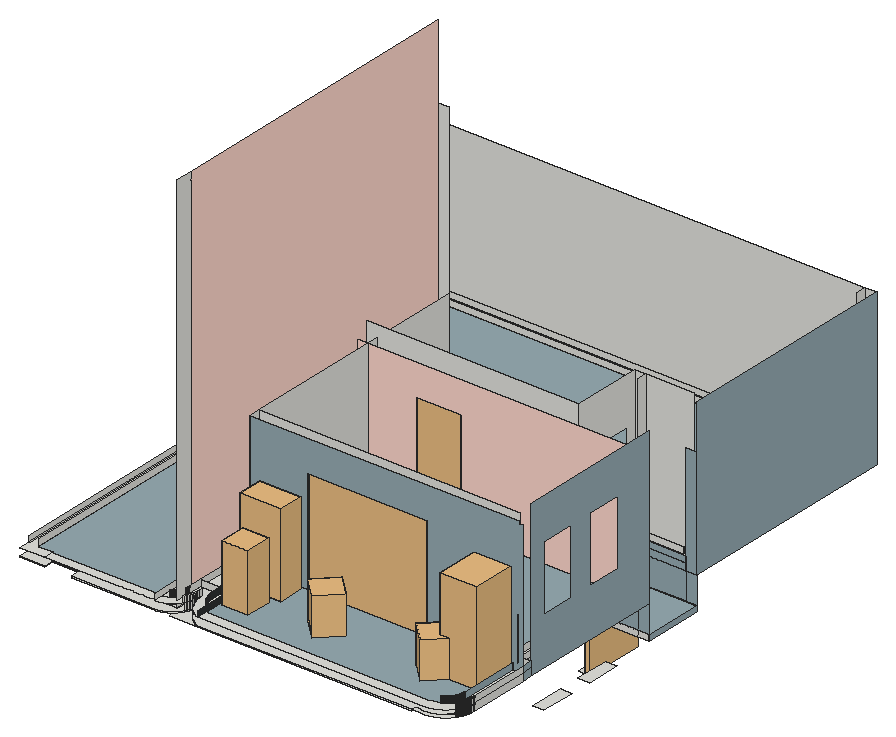
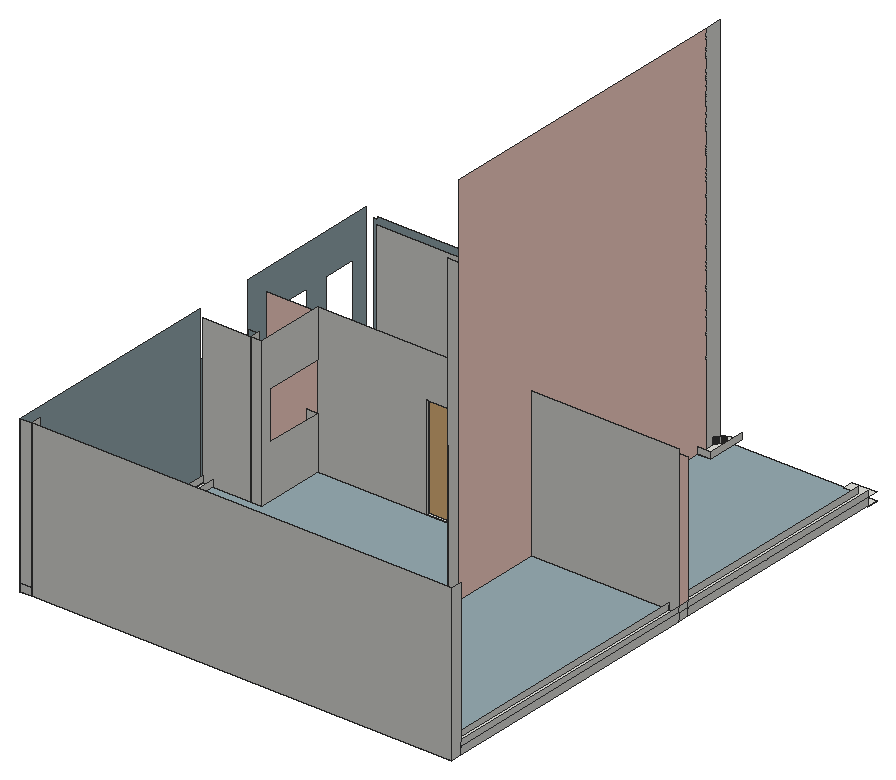
# SketchUp Ruby script. Lengths in inches.
U = 1.inch
M = Sketchup.active_model
def pt(a) = Geom::Point3d.new(a.map { |v| v * U })
def face(e, loops, mat)
  f = e.add_face(loops[0].map { |a| pt(a) })
  loops[1..].each { |l| e.add_face(l.map { |a| pt(a) }).erase! }
  f.material = f.back_material = mat if mat
  f
end
# faces: each face lists its corners as indices into pts; further lists are holes
def faces(e, pts, list, mat = nil) = list.each { |f| face(e, (f[0].is_a?(Array) ? f : [f]).map { |l| l.map { |i| pts[i] } }, mat) }
# xy, xz, yz: faces in a plane at the given z, y or x. An outline is a flat list of corners, or four numbers for a rectangle; further outlines are holes
def ring(l) = l.size == 4 ? [[l[0], l[1]], [l[2], l[1]], [l[2], l[3]], [l[0], l[3]]] : l.each_slice(2).to_a
def flat(e, list, mat, &to3) = list.each { |f| face(e, (f[0].is_a?(Array) ? f : [f]).map { |l| ring(l).map { |u, v| to3.(u, v) } }, mat) }
def xy(e, z, list, mat = nil) = flat(e, list, mat) { |x, y| [x, y, z] }
def xz(e, y, list, mat = nil) = flat(e, list, mat) { |x, z| [x, y, z] }
def yz(e, x, list, mat = nil) = flat(e, list, mat) { |y, z| [x, y, z] }
def lines(e, pts, list) = list.each { |a, b| e.add_line(pt(pts[a]), pt(pts[b])) }
# prism: a flat outline (further loops are holes) pulled along v
def prism(e, loops, v, mat = nil)
  f = face(e, loops, mat); d = Geom::Vector3d.new(v.map { |x| x * U })
  f.pushpull(f.normal.samedirection?(d) ? d.length : -d.length)
end
def box(e, o, s, mat = nil) = prism(e, [[o, [o[0] + s[0], o[1], o[2]], [o[0] + s[0], o[1] + s[1], o[2]], [o[0], o[1] + s[1], o[2]]]], [0, 0, s[2]], mat)
def at(x, y, z, deg = 0) = Geom::Transformation.translation(pt([x, y, z])) * Geom::Transformation.rotation(ORIGIN, Z_AXIS, deg.degrees)
def axes(o, x, y, z) = Geom::Transformation.new([*x, 0, *y, 0, *z, 0, *pt(o).to_a, 1])
def part(name) = M.definitions.add(name)
# library, detail: a bought-in or finely detailed component or shape, given as its bounding box
def library(name, o, s) = part(name).tap { |d| box(d.entities, o, s) }
def detail(e, o, s) = box(e.add_group.entities, o, s)
def put(e, d, t, mat = nil) = e.add_instance(d, t).tap { |i| i.material = mat if mat }
def group(e, t, mat = nil) = e.add_group.tap { |g| g.transformation = t; g.material = mat if mat }.entities
root = M.entities
M.materials.add("Generic").color = [150, 171, 178]
M.materials.add("Generic\#1").color = [47, 50, 50]
M.materials.add("[Color B01]").color = [255, 216, 204]
M.materials.add("[Color M00]").color = [207, 192, 171]
M.materials.add("[Color M07]").color = [58, 58, 58]
c1 = library("Tlon Light 650 Ceiling 152 007",[-12.8,-12.8,-3.78],[25.6,25.6,3.58])
c2 = library("Potted Plant 60-25",[-10.7,-10.47,0],[21.2,21.27,47.12])
c3 = library("Chair 288 019",[-10.59,-11.4,0],[21.2,22.8,30.25])
c4 = library("Potted Plant 02",[-16.98,-19.78,0],[30.04,38.68,37.52])
c5 = library("Plant 260 020",[-18.86,-7.03,0.01],[33.61,20.04,67.26])
c6 = library("Window 46-47",[-61.02,-2.17,0],[122.04,4.34,74.02])
c7 = library("Door 109 063",[-20.08,-3.39,-0.2],[40.16,6.85,82.67])
c8 = library("Window 46-06",[-34.91,-2.12,0],[69.82,4.27,59.06])
xy(root,170.836,[[230.012,233.0625,272.45,234.0625]],"[Color M07]")
xy(root,172.965,[[232.141,233.0625,270.321,233.662]],"[Color M07]")
xy(root,177.1,[[304.218,243.0625,313.218,291.0625]])
xy(root,195.896,[[232.141,233.0625,270.321,233.662]],"[Color M07]")
xy(root,198.024,[[230.012,233.0625,272.45,234.0625]],"[Color M07]")
xy(root,210,[[187.218,114.0625,283.218,123.0625],[179.03,234.0625,215.03,243.0625]])
xy(root,215.248,[[304.218,243.0625,313.218,291.0625]],"Generic")
xy(root,215.411,[[352.218,136.159,361.218,164.284],[352.218,182.159,361.218,210.284]])
xy(root,219.122,[[313.218,243.0625,361.405,291.0625]],"Generic")
xy(root,223.737,[[313.218,243.0625,361.405,291.0625]],"Generic")
xy(root,245,[[10.218,42.0625,10.218,51.0625,130.218,51.0625,130.218,123.0625,139.218,123.0625,139.218,114.0625,357.218,114.0625,357.218,70.0625,357.274,69.418,357.311,68.771,357.329,68.124,357.328,67.477,357.307,66.83,357.268,66.184,357.209,65.54,357.132,64.897,357.035,64.257,356.92,63.62,356.786,62.987,356.633,62.358,356.461,61.734,356.272,61.115,356.064,60.502,355.838,59.895,355.594,59.296,355.332,58.704,355.054,58.119,354.758,57.544,354.445,56.977,354.115,56.42,353.769,55.873,353.408,55.336,353.03,54.811,352.637,54.296,352.229,53.794,351.806,53.303,351.37,52.826,350.919,52.361,350.454,51.911,349.977,51.474,349.486,51.051,348.984,50.643,348.47,50.25,347.944,49.873,347.407,49.511,346.86,49.165,346.303,48.835,345.736,48.523,345.161,48.227,344.576,47.948,343.984,47.686,343.385,47.442,342.778,47.216,342.165,47.009,341.546,46.819,340.922,46.647,340.293,46.495,339.66,46.36,339.023,46.245,338.383,46.148,337.741,46.071,337.096,46.012,336.45,45.973,335.803,45.953,335.156,45.951,334.509,45.969,333.862,46.006,333.218,46.0625,328.648,46.0625,328.648,42.0625,154.672,42.0625,152.46,43.109,150.36,44.367,148.394,45.823,146.578,47.464,144.932,49.275,143.47,51.238,142.207,53.333,141.154,55.543,140.322,57.844,139.718,60.216,139.349,62.635,139.218,65.078,139.218,63.384,139.2,62.851,139.107,61.74,138.959,60.636,138.756,59.54,138.498,58.456,138.186,57.387,137.82,56.334,137.402,55.301,136.933,54.29,136.414,53.304,135.846,52.346,135.231,51.417,134.57,50.52,133.865,49.657,133.117,48.831,132.329,48.043,131.502,47.296,130.639,46.592,129.741,45.931,128.812,45.317,127.853,44.749,126.867,44.231,125.856,43.763,124.822,43.346,123.769,42.981,122.699,42.67,121.615,42.412,120.52,42.21,119.415,42.0625,51.935,42.0625,51.935,50.129,29.81,50.129,29.81,42.0625],[131.803,42.0625,131.538,42.727,130.991,44.637,130.639,46.592,131.502,47.296,132.329,48.043,133.117,48.831,133.865,49.657,134.57,50.52,135.231,51.417,135.846,52.346,136.414,53.304,136.933,54.29,137.402,55.301,137.82,56.334,138.186,57.387,138.498,58.456,138.756,59.54,138.959,60.636,139.107,61.74,139.2,62.851,139.218,63.384,139.237,63.964,139.218,65.078,139.349,62.635,139.718,60.216,140.322,57.844,141.154,55.543,142.207,53.333,143.47,51.238,144.932,49.275,146.578,47.464,148.394,45.823,150.36,44.367,152.46,43.109,154.672,42.0625]])
xy(root,246,[[10.218,42.0625,29.81,42.0625,29.81,50.129,51.935,50.129,51.935,42.0625,119.415,42.0625,120.52,42.21,121.615,42.412,122.699,42.67,123.769,42.981,124.822,43.346,125.856,43.763,126.867,44.231,127.853,44.749,128.812,45.317,129.741,45.931,130.639,46.592,131.502,47.296,132.329,48.043,133.117,48.831,133.865,49.657,134.57,50.52,135.231,51.417,135.846,52.346,136.414,53.304,136.933,54.29,137.402,55.301,137.82,56.334,138.186,57.387,138.498,58.456,138.756,59.54,138.959,60.636,139.107,61.74,139.2,62.851,139.218,63.384,139.218,65.078,139.349,62.635,139.718,60.216,140.322,57.844,141.154,55.543,142.207,53.333,143.47,51.238,144.932,49.275,146.578,47.464,148.394,45.823,150.36,44.367,152.46,43.109,154.672,42.0625,328.648,42.0625,328.648,46.0625,333.218,46.0625,333.862,46.006,334.509,45.969,335.156,45.951,335.803,45.953,336.45,45.973,337.096,46.012,337.741,46.071,338.383,46.148,339.023,46.245,339.66,46.36,340.293,46.495,340.922,46.647,341.546,46.819,342.165,47.009,342.778,47.216,343.385,47.442,343.984,47.686,344.576,47.948,345.161,48.227,345.736,48.523,346.303,48.835,346.86,49.165,347.407,49.511,347.944,49.873,348.47,50.25,348.984,50.643,349.486,51.051,349.977,51.474,350.454,51.911,350.919,52.361,351.37,52.826,351.806,53.303,352.229,53.794,352.637,54.296,353.03,54.811,353.408,55.336,353.769,55.873,354.115,56.42,354.445,56.977,354.758,57.544,355.054,58.119,355.332,58.704,355.594,59.296,355.838,59.895,356.064,60.502,356.272,61.115,356.461,61.734,356.633,62.358,356.786,62.987,356.92,63.62,357.035,64.257,357.132,64.897,357.209,65.54,357.268,66.184,357.307,66.83,357.328,67.477,357.329,68.124,357.311,68.771,357.274,69.418,357.218,70.0625,357.218,114.0625,139.218,114.0625,139.218,123.0625,130.218,123.0625,130.218,51.0625,10.218,51.0625],[328.648,42.0625,337.222,42.0625,339.638,42.186,339.726,42.194,340.35,42.268,340.972,42.358,341.591,42.464,342.207,42.587,342.82,42.726,343.429,42.88,344.034,43.051,344.634,43.237,345.229,43.439,345.818,43.657,346.402,43.889,346.979,44.137,347.55,44.4,348.113,44.678,348.669,44.971,349.218,45.278,349.758,45.599,350.289,45.934,350.811,46.283,351.324,46.646,351.828,47.022,352.321,47.411,352.804,47.813,353.277,48.227,353.738,48.654,354.188,49.092,354.627,49.542,355.053,50.003,355.467,50.476,355.869,50.959,356.258,51.452,356.634,51.956,356.997,52.469,357.346,52.991,357.681,53.523,358.002,54.0625,358.309,54.611,358.602,55.167,358.88,55.73,359.143,56.301,359.391,56.878,359.624,57.462,359.841,58.051,360.043,58.646,360.229,59.246,360.4,59.851,360.554,60.46,360.693,61.073,360.816,61.689,360.922,62.308,361.012,62.93,361.086,63.554,361.094,63.642,361.218,66.0625,361.218,114.0625,357.218,114.0625,357.218,70.0625,357.274,69.418,357.311,68.771,357.329,68.124,357.328,67.477,357.307,66.83,357.268,66.184,357.209,65.54,357.132,64.897,357.035,64.257,356.92,63.62,356.786,62.987,356.633,62.358,356.461,61.734,356.272,61.115,356.064,60.502,355.838,59.895,355.594,59.296,355.332,58.704,355.054,58.119,354.758,57.544,354.445,56.977,354.115,56.42,353.769,55.873,353.408,55.336,353.03,54.811,352.637,54.296,352.229,53.794,351.806,53.303,351.37,52.826,350.919,52.361,350.454,51.911,349.977,51.474,349.486,51.051,348.984,50.643,348.47,50.25,347.944,49.873,347.407,49.511,346.86,49.165,346.303,48.835,345.736,48.523,345.161,48.227,344.576,47.948,343.984,47.686,343.385,47.442,342.778,47.216,342.165,47.009,341.546,46.819,340.922,46.647,340.293,46.495,339.66,46.36,339.023,46.245,338.383,46.148,337.741,46.071,337.096,46.012,336.45,45.973,335.803,45.953,335.156,45.951,334.509,45.969,333.862,46.006,333.218,46.0625,328.648,46.0625],[10.218,51.0625,10.218,234.0625,130.218,234.0625,130.218,65.078,130.098,63.249,129.74,61.451,129.151,59.715,128.34,58.07,127.321,56.546,126.112,55.168,124.734,53.959,123.21,52.94,121.565,52.129,119.829,51.54,118.031,51.182,116.202,51.0625],[116.202,51.0625,118.031,51.182,119.829,51.54,121.565,52.129,123.21,52.94,124.734,53.959,126.112,55.168,127.321,56.546,128.34,58.07,129.151,59.715,129.74,61.451,130.098,63.249,130.218,65.078,130.218,51.0625],[361.094,63.642,361.144,64.179,361.185,64.806,361.209,65.434,361.218,66.0625],
  [139.218,114.0625,361.218,123.0625],[130.218,123.0625,139.218,234.0625],[139.218,123.0625,352.218,234.0625],[352.218,123.0625,361.218,243.0625],[10.218,234.0625,130.218,243.0625],
  [130.218,234.0625,139.218,243.0625],[139.218,234.0625,352.218,243.0625],[10.218,243.0625,10.218,465.0625,352.218,465.0625,352.218,300.0625,304.218,300.0625,304.218,243.0625,139.218,243.0625,139.218,317.038,130.218,317.038,130.218,243.0625],[130.218,243.0625,139.218,317.038],[304.218,243.0625,313.218,300.0625],
  [313.218,291.0625,352.218,300.0625],[352.218,291.0625,361.218,474.0625],[10.218,465.0625,352.218,474.0625]])
xy(root,252,[[10.218,42.0625,10.218,465.0625,352.218,465.0625,352.218,291.0625,313.218,291.0625,313.218,243.0625,352.218,243.0625,352.218,123.0625,361.218,123.0625,361.218,66.0625,361.209,65.434,361.185,64.806,361.144,64.179,361.094,63.642,361.086,63.17,361.031,62.701,360.967,62.234,360.893,61.768,360.81,61.304,360.718,60.841,360.617,60.381,360.506,59.922,360.387,59.466,360.258,59.012,360.12,58.561,359.973,58.113,359.818,57.668,359.653,57.226,359.48,56.787,359.298,56.352,359.107,55.921,358.908,55.494,358.701,55.07,358.484,54.651,358.26,54.236,358.027,53.826,357.787,53.421,357.538,53.02,357.281,52.624,357.016,52.234,356.744,51.849,356.464,51.47,356.176,51.096,355.881,50.728,355.579,50.366,355.27,50.01,354.953,49.66,354.63,49.317,354.3,48.98,353.963,48.65,353.62,48.327,353.27,48.01,352.914,47.701,352.552,47.399,352.184,47.104,351.81,46.816,351.431,46.536,351.046,46.264,350.656,45.999,350.26,45.742,349.859,45.494,349.454,45.253,349.044,45.02,348.629,44.796,348.21,44.58,347.786,44.372,347.359,44.173,346.928,43.982,346.493,43.8,346.054,43.627,345.612,43.462,345.167,43.307,344.719,43.16,344.268,43.022,343.814,42.893,343.358,42.774,342.899,42.663,342.439,42.562,341.976,42.47,341.512,42.387,341.046,42.313,340.579,42.249,340.111,42.194,339.638,42.186,339.101,42.136,338.474,42.095,337.846,42.071,337.222,42.0625,154.672,42.0625,154.672,51.212,154.844,51.084,156.266,50.232,156.484,50.129,337.165,50.129,337.635,50.135,338.051,50.152,338.468,50.179,339.198,50.246,339.567,50.253,339.867,50.294,340.174,50.342,340.479,50.397,340.784,50.458,341.087,50.524,341.389,50.597,341.69,50.676,341.988,50.761,342.286,50.851,342.581,50.948,342.874,51.05,343.165,51.159,343.454,51.273,343.74,51.393,344.024,51.518,344.306,51.65,344.585,51.786,344.861,51.929,345.134,52.076,345.404,52.23,345.671,52.388,345.935,52.552,346.196,52.721,346.453,52.896,346.706,53.075,346.956,53.259,347.202,53.449,347.445,53.643,347.683,53.842,347.917,54.046,348.148,54.254,348.374,54.467,348.596,54.684,348.813,54.906,349.026,55.132,349.234,55.363,349.438,55.597,349.637,55.836,349.831,56.078,350.021,56.324,350.205,56.574,350.385,56.828,350.559,57.085,350.728,57.345,350.892,57.609,351.05,57.876,351.204,58.146,351.351,58.419,351.494,58.695,351.631,58.974,351.762,59.256,351.887,59.54,352.007,59.826,352.121,60.115,352.23,60.406,352.332,60.699,352.429,60.995,352.519,61.292,352.604,61.59,352.683,61.891,352.756,62.193,352.823,62.496,352.883,62.801,352.938,63.106,352.986,63.413,353.028,63.713,353.034,64.082,353.101,64.8125,353.128,65.229,353.145,65.645,353.151,66.115,353.151,114.996,344.151,114.996,344.151,234.996,305.151,234.996,305.151,299.129,344.151,299.129,344.151,456.996,18.284,456.996,18.284,50.129,29.81,50.129,29.81,42.0625],[119.415,42.0625,119.415,50.209,119.95,50.308,120.64,50.472,121.321,50.67,121.991,50.902,122.649,51.167,123.293,51.466,123.921,51.796,124.531,52.157,125.123,52.548,125.694,52.968,126.244,53.417,126.77,53.893,127.272,54.394,127.748,54.92,128.197,55.469,128.618,56.04,129.009,56.632,129.371,57.242,129.701,57.87,130,58.513,130.266,59.171,130.499,59.841,130.697,60.522,130.862,61.212,130.991,61.909,131.085,62.612,131.144,63.319,131.151,63.517,131.151,74.3125,146.799,74.3125,147.383,63.462,147.633,61.823,148.042,60.216,148.606,58.657,149.319,57.16,150.175,55.74,151.166,54.41,152.281,53.183,153.511,52.071,154.672,51.212,154.672,42.0625,152.46,43.109,150.36,44.367,148.394,45.823,146.578,47.464,144.932,49.275,143.47,51.238,142.207,53.333,141.154,55.543,140.322,57.844,139.718,60.216,139.349,62.635,139.218,65.078,139.218,63.384,139.2,62.851,139.107,61.74,138.959,60.636,138.756,59.54,138.498,58.456,138.186,57.387,137.82,56.334,137.402,55.301,136.933,54.29,136.414,53.304,135.846,52.346,135.231,51.417,134.57,50.52,133.865,49.657,133.117,48.831,132.329,48.043,131.502,47.296,130.639,46.592,129.741,45.931,128.812,45.317,127.853,44.749,126.867,44.231,125.856,43.763,124.822,43.346,123.769,42.981,122.699,42.67,121.615,42.412,120.52,42.21],[119.415,50.209,119.415,74.3125,131.151,74.3125,131.151,63.517,131.144,63.319,131.085,62.612,130.991,61.909,130.862,61.212,130.697,60.522,130.499,59.841,130.266,59.171,130,58.513,129.701,57.87,129.371,57.242,129.009,56.632,128.618,56.04,128.197,55.469,127.748,54.92,127.272,54.394,126.77,53.893,126.244,53.417,125.694,52.968,125.123,52.548,124.531,52.157,123.921,51.796,123.293,51.466,122.649,51.167,121.991,50.902,121.321,50.67,120.64,50.472,119.95,50.308],[154.672,51.212,153.511,52.071,152.281,53.183,151.166,54.41,150.175,55.74,149.319,57.16,148.606,58.657,148.042,60.216,147.633,61.823,147.383,63.462,146.799,74.3125,154.672,74.3125],[139.218,63.384,139.218,65.078,139.237,63.964],
  [131.151,74.3125,131.151,365.116,146.799,74.3125],[187.218,114.0625,283.218,123.0625],[179.03,234.0625,215.03,243.0625]])
xy(root,252,[[[18.284,50.129,118.879,50.129,119.252,50.179,119.415,50.209,119.415,74.3125,131.151,74.3125,131.151,365.116,146.799,74.3125,154.672,74.3125,154.672,51.212,154.844,51.084,156.266,50.232,156.484,50.129,337.165,50.129,337.635,50.135,338.051,50.152,338.468,50.179,339.198,50.246,339.567,50.253,339.867,50.294,340.174,50.342,340.479,50.397,340.784,50.458,341.087,50.524,341.389,50.597,341.69,50.676,341.988,50.761,342.286,50.851,342.581,50.948,342.874,51.05,343.165,51.159,343.454,51.273,343.74,51.393,344.024,51.518,344.306,51.65,344.585,51.786,344.861,51.929,345.134,52.076,345.404,52.23,345.671,52.388,345.935,52.552,346.196,52.721,346.453,52.896,346.706,53.075,346.956,53.259,347.202,53.449,347.445,53.643,347.683,53.842,347.917,54.046,348.148,54.254,348.374,54.467,348.596,54.684,348.813,54.906,349.026,55.132,349.234,55.363,349.438,55.597,349.637,55.836,349.831,56.078,350.021,56.324,350.205,56.574,350.385,56.828,350.559,57.085,350.728,57.345,350.892,57.609,351.05,57.876,351.204,58.146,351.351,58.419,351.494,58.695,351.631,58.974,351.762,59.256,351.887,59.54,352.007,59.826,352.121,60.115,352.23,60.406,352.332,60.699,352.429,60.995,352.519,61.292,352.604,61.59,352.683,61.891,352.756,62.193,352.823,62.496,352.883,62.801,352.938,63.106,352.986,63.413,353.028,63.713,353.034,64.082,353.101,64.8125,353.128,65.229,353.145,65.645,353.151,66.115,353.151,114.996,344.151,114.996,344.151,234.996,305.151,234.996,305.151,299.129,344.151,299.129,344.151,456.996,18.284,456.996],[187.218,114.0625,283.218,123.0625],[179.03,234.0625,215.03,243.0625]]],"Generic")
xz(root,74.3125,[[119.415,252,154.672,257]])
xz(root,114.0625,[[139.218,245,357.218,246]])
xz(root,114.0625,[[[139.218,246,361.218,246,361.218,360,358.218,360,358.218,362,139.218,362],[187.218,252,283.218,336],[356.352,257,356.352,293,355.796,293,355.796,294,358.484,294,358.484,293,358.109,293,358.109,257]]],"Generic")
xz(root,114.996,[[344.151,252,353.151,257]])
xz(root,123.0625,[[130.218,245,139.218,246],[[139.218,246,352.218,362],[187.218,252,283.218,336]],[352.218,246,361.218,252],[352.218,252,361.218,257]])
xz(root,233.0625,[[[230.012,170.836,272.45,198.024],[232.141,172.965,270.321,195.896]]],"[Color M07]")
xz(root,233.662,[[232.141,172.965,270.321,195.896]],"[Color M00]")
xz(root,234.0625,[[[10.218,246,352.218,362],[179.03,252,215.03,336]]],"[Color B01]")
xz(root,234.996,[[305.151,252,344.151,257]])
xz(root,243.0625,[[304.218,215.248,304.218,246,313.218,246,313.218,223.737,352.218,223.737,352.218,219.122,313.218,219.122,313.218,215.248],[352.218,219.122,361.218,223.737],[361.218,219.122,361.405,223.737],[[10.218,246,304.218,372],[179.03,252,215.03,336]],[304.218,246,313.218,294.452]])
xz(root,243.0625,[[313.218,223.737,352.218,246],[352.218,223.737,361.218,246],[313.218,246,352.218,252],[352.218,246,361.218,335.818],[313.218,252,352.218,257]],"Generic")
xz(root,291.0625,[[304.218,177.1,313.218,215.248],[313.218,219.122,352.218,223.737],[352.218,219.122,361.218,223.737],[361.218,219.122,361.405,223.737]])
xz(root,291.0625,[[313.218,223.737,352.218,246],[352.218,223.737,361.218,246],[313.218,246,352.218,252],[352.218,246,361.218,335.818],[313.218,252,352.218,257]],"Generic")
xz(root,299.129,[[305.151,252,344.151,257]])
xz(root,300.0625,[[304.218,246,313.218,372],[313.218,246,352.218,372]])
xz(root,317.038,[[130.218,246,139.218,498]])
xz(root,456.996,[[18.284,252,344.151,257]])
xz(root,465.0625,[[10.218,246,352.218,252],[10.218,252,352.218,257]])
xz(root,474.0625,[[10.218,246,352.218,372],[352.218,246,361.218,252],[352.218,252,361.218,372]])
yz(root,10.218,[[51.0625,246,234.0625,252],[234.0625,246,243.0625,252],[243.0625,246,465.0625,252],[465.0625,246,474.0625,372],[51.0625,252,234.0625,257],
  [234.0625,252,243.0625,257],[243.0625,252,465.0625,257]])
yz(root,18.284,[[51.0625,252,234.0625,257],[234.0625,252,243.0625,257],[243.0625,252,456.996,257]])
yz(root,119.415,[[42.0625,252,74.3125,257]])
yz(root,130.218,[[51.0625,245,65.078,246],[65.078,245,123.0625,246],[51.0625,246,65.078,558]])
yz(root,130.218,[[65.078,246,317.038,558]],"[Color B01]")
yz(root,131.151,[[63.517,252,365.116,257]])
yz(root,139.218,[[63.384,245,65.078,246],[114.0625,245,123.0625,246],[63.384,246,65.078,252],[114.0625,246,123.0625,362],[123.0625,246,317.038,362],
  [63.384,252,65.078,257]])
yz(root,154.672,[[42.0625,252,74.3125,257]],"Generic\#1")
yz(root,179.03,[[234.0625,252,243.0625,336]])
yz(root,187.218,[[114.0625,252,123.0625,336]])
yz(root,215.03,[[234.0625,252,243.0625,336]])
yz(root,230.012,[[233.0625,170.836,234.0625,198.024]],"[Color M07]")
yz(root,232.141,[[233.0625,172.965,233.662,195.896]],"[Color M07]")
yz(root,270.321,[[233.0625,172.965,233.662,195.896]],"[Color M07]")
yz(root,272.45,[[233.0625,170.836,234.0625,198.024]],"[Color M07]")
yz(root,283.218,[[114.0625,252,123.0625,336]])
yz(root,304.218,[[243.0625,246,243.0625,294.452,291.0625,294.452,291.0625,333.326,243.0625,333.326,243.0625,372,300.0625,372,300.0625,246]])
yz(root,305.151,[[234.996,252,299.129,257]])
yz(root,313.218,[[291.0625,246,300.0625,372]])
yz(root,313.218,[[243.0625,215.248,291.0625,219.122],[243.0625,223.737,291.0625,246],[243.0625,246,291.0625,252],[243.0625,252,291.0625,257]],"Generic")
yz(root,344.151,[[114.996,252,234.0625,257],[234.0625,252,234.996,257],[299.129,252,300.0625,257],[300.0625,252,456.996,257]])
yz(root,352.218,[[123.0625,246,234.0625,252],[234.0625,246,243.0625,252],[291.0625,246,300.0625,252],[300.0625,246,465.0625,252],[465.0625,246,474.0625,372],
  [123.0625,252,234.0625,257],[234.0625,252,243.0625,257],[291.0625,252,300.0625,257],[300.0625,252,465.0625,257]])
yz(root,353.151,[[114.0625,252,114.996,257]])
yz(root,353.151,[[66.115,252,114.0625,257]],"Generic")
yz(root,357.218,[[70.0625,245,114.0625,246]])
yz(root,361.218,[[66.0625,246,114.0625,252],[66.0625,252,114.0625,257]])
yz(root,361.218,[[114.0625,246,123.0625,252],[[123.0625,246,243.0625,372],[135.565,285.591,163.627,338.859],[182.69,285.591,210.752,338.859]],[291.0625,246,474.0625,372],[114.0625,252,123.0625,257]],"Generic")
yz(root,361.405,[[243.0625,219.122,291.0625,223.737]],"Generic")
p = [[142.207,53.333,245],[142.207,53.333,246],[143.47,51.238,246],[143.47,51.238,245],[350.454,51.911,246],[350.919,52.361,246],
  [350.919,52.361,245],[350.454,51.911,245],[135.846,52.346,245],[135.846,52.346,246],[136.414,53.304,246],[136.414,53.304,245],
  [351.37,52.826,246],[351.37,52.826,245],[351.806,53.303,246],[351.806,53.303,245],[136.933,54.29,246],[136.933,54.29,245],
  [141.154,55.543,245],[141.154,55.543,246],[352.229,53.794,246],[352.229,53.794,245],[352.637,54.296,246],[352.637,54.296,245],
  [137.402,55.301,246],[137.402,55.301,245],[353.03,54.811,246],[353.03,54.811,245],[353.408,55.336,246],[353.408,55.336,245],
  [137.82,56.334,246],[137.82,56.334,245],[353.769,55.873,246],[353.769,55.873,245],[140.322,57.844,245],[140.322,57.844,246],
  [354.115,56.42,246],[354.115,56.42,245],[138.186,57.387,246],[138.186,57.387,245],[354.445,56.977,246],[354.445,56.977,245],
  [354.758,57.544,246],[354.758,57.544,245],[138.498,58.456,246],[138.498,58.456,245],[355.054,58.119,246],[355.054,58.119,245],
  [139.718,60.216,245],[139.718,60.216,246],[355.332,58.704,246],[355.332,58.704,245],[138.756,59.54,246],[138.756,59.54,245],
  [355.594,59.296,246],[355.594,59.296,245],[355.838,59.895,246],[355.838,59.895,245],[138.959,60.636,246],[138.959,60.636,245],
  [356.064,60.502,246],[356.064,60.502,245],[139.349,62.635,245],[139.349,62.635,246],[356.272,61.115,246],[356.272,61.115,245],
  [139.107,61.74,246],[139.107,61.74,245],[356.461,61.734,246],[356.461,61.734,245],[139.2,62.851,246],[139.2,62.851,245],
  [356.633,62.358,246],[356.633,62.358,245],[356.786,62.987,246],[356.786,62.987,245],[139.218,65.078,245],[139.218,65.078,246],
  [139.218,63.384,246],[139.218,63.384,245],[356.92,63.62,246],[356.92,63.62,245],[139.237,63.964,246],[139.237,63.964,245],
  [357.035,64.257,246],[357.035,64.257,245],[357.132,64.897,246],[357.132,64.897,245],[357.209,65.54,246],[357.209,65.54,245],
  [357.268,66.184,246],[357.268,66.184,245],[357.307,66.83,246],[357.307,66.83,245],[357.328,67.477,246],[357.328,67.477,245],
  [357.329,68.124,246],[357.329,68.124,245],[357.311,68.771,246],[357.311,68.771,245],[357.274,69.418,246],[357.274,69.418,245],
  [357.218,70.0625,246],[357.218,70.0625,245],[142.207,53.333,252],[143.47,51.238,252],[356.744,51.849,246],[357.016,52.234,246],
  [357.016,52.234,252],[356.744,51.849,252],[357.281,52.624,246],[357.281,52.624,252],[135.846,52.346,252],[136.414,53.304,252],
  [357.538,53.02,246],[357.538,53.02,252],[357.787,53.421,246],[357.787,53.421,252],[136.933,54.29,252],[141.154,55.543,252],
  [358.027,53.826,246],[358.027,53.826,252],[358.26,54.236,246],[358.26,54.236,252],[358.484,54.651,246],[358.484,54.651,252],
  [137.402,55.301,252],[358.701,55.07,246],[358.701,55.07,252],[358.908,55.494,246],[358.908,55.494,252],[137.82,56.334,252],
  [140.322,57.844,252],[359.107,55.921,246],[359.107,55.921,252],[359.298,56.352,246],[359.298,56.352,252],[138.186,57.387,252],
  [359.48,56.787,246],[359.48,56.787,252],[359.653,57.226,246],[359.653,57.226,252],[359.818,57.668,246],[359.818,57.668,252],
  [138.498,58.456,252],[359.973,58.113,246],[359.973,58.113,252],[139.718,60.216,252],[360.12,58.561,246],[360.12,58.561,252],
  [138.756,59.54,252],[360.258,59.012,246],[360.258,59.012,252],[360.387,59.466,246],[360.387,59.466,252],[138.959,60.636,252],
  [360.506,59.922,246],[360.506,59.922,252],[360.617,60.381,246],[360.617,60.381,252],[139.349,62.635,252],[360.718,60.841,246],
  [360.718,60.841,252],[139.107,61.74,252],[360.81,61.304,246],[360.81,61.304,252],[360.893,61.768,246],[360.893,61.768,252],
  [139.2,62.851,252],[360.967,62.234,246],[360.967,62.234,252],[361.031,62.701,246],[361.031,62.701,252],[139.218,65.078,252],
  [361.086,63.17,246],[361.086,63.17,252],[139.218,63.384,252],[361.094,63.642,246],[361.094,63.642,252],[139.237,63.964,252],
  [361.144,64.179,246],[361.144,64.179,252],[361.185,64.806,246],[361.185,64.806,252],[361.209,65.434,246],[361.209,65.434,252],
  [361.218,66.0625,246],[361.218,66.0625,252],[142.207,53.333,257],[143.47,51.238,257],[135.231,51.417,252],[135.231,51.417,257],
  [135.846,52.346,257],[124.531,52.157,252],[123.921,51.796,252],[123.921,51.796,257],[124.531,52.157,257],[357.016,52.234,257],
  [356.744,51.849,257],[345.134,52.076,252],[344.861,51.929,252],[344.861,51.929,257],[345.134,52.076,257],[153.511,52.071,252],
  [152.281,53.183,252],[152.281,53.183,257],[153.511,52.071,257],[345.404,52.23,252],[345.404,52.23,257],[125.123,52.548,252],
  [125.123,52.548,257],[345.671,52.388,252],[345.671,52.388,257],[357.281,52.624,257],[136.414,53.304,257],[345.935,52.552,252],
  [345.935,52.552,257],[125.694,52.968,252],[125.694,52.968,257],[346.196,52.721,252],[346.196,52.721,257],[357.538,53.02,257],
  [346.453,52.896,252],[346.453,52.896,257],[346.706,53.075,252],[346.706,53.075,257],[126.244,53.417,252],[126.244,53.417,257],
  [357.787,53.421,257],[346.956,53.259,252],[346.956,53.259,257],[151.166,54.41,252],[151.166,54.41,257],[136.933,54.29,257],
  [141.154,55.543,257],[347.202,53.449,252],[347.202,53.449,257],[126.77,53.893,252],[126.77,53.893,257],[347.445,53.643,252],
  [347.445,53.643,257],[358.027,53.826,257],[347.683,53.842,252],[347.683,53.842,257],[347.917,54.046,252],[347.917,54.046,257],
  [358.26,54.236,257],[127.272,54.394,252],[127.272,54.394,257],[348.148,54.254,252],[348.148,54.254,257],[358.484,54.651,257],
  [137.402,55.301,257],[348.374,54.467,252],[348.374,54.467,257],[127.748,54.92,252],[127.748,54.92,257],[150.175,55.74,252],
  [150.175,55.74,257],[348.596,54.684,252],[348.596,54.684,257],[348.813,54.906,252],[348.813,54.906,257],[358.701,55.07,257],
  [128.197,55.469,252],[128.197,55.469,257],[349.026,55.132,252],[349.026,55.132,257],[349.234,55.363,252],[349.234,55.363,257],
  [358.908,55.494,257],[137.82,56.334,257],[349.438,55.597,252],[349.438,55.597,257],[128.618,56.04,252],[128.618,56.04,257],
  [140.322,57.844,257],[359.107,55.921,257],[349.637,55.836,252],[349.637,55.836,257],[149.319,57.16,252],[149.319,57.16,257],
  [349.831,56.078,252],[349.831,56.078,257],[359.298,56.352,257],[129.009,56.632,252],[129.009,56.632,257],[350.021,56.324,252],
  [350.021,56.324,257],[138.186,57.387,257],[350.205,56.574,252],[350.205,56.574,257],[359.48,56.787,257],[129.371,57.242,252],
  [129.371,57.242,257],[350.385,56.828,252],[350.385,56.828,257],[350.559,57.085,252],[350.559,57.085,257],[359.653,57.226,257],
  [350.728,57.345,252],[350.728,57.345,257],[129.701,57.87,252],[129.701,57.87,257],[148.606,58.657,252],[148.606,58.657,257],
  [359.818,57.668,257],[350.892,57.609,252],[350.892,57.609,257],[138.498,58.456,257],[351.05,57.876,252],[351.05,57.876,257],
  [359.973,58.113,257],[139.718,60.216,257],[130,58.513,252],[130,58.513,257],[351.204,58.146,252],[351.204,58.146,257],
  [351.351,58.419,252],[351.351,58.419,257],[360.12,58.561,257],[351.494,58.695,252],[351.494,58.695,257],[130.266,59.171,252],
  [130.266,59.171,257],[138.756,59.54,257],[360.258,59.012,257],[148.042,60.216,252],[148.042,60.216,257],[351.631,58.974,252],
  [351.631,58.974,257],[351.762,59.256,252],[351.762,59.256,257],[360.387,59.466,257],[130.499,59.841,252],[130.499,59.841,257],
  [351.887,59.54,252],[351.887,59.54,257],[138.959,60.636,257],[352.007,59.826,252],[352.007,59.826,257],[360.506,59.922,257],
  [130.697,60.522,252],[130.697,60.522,257],[352.121,60.115,252],[352.121,60.115,257],[360.617,60.381,257],[352.23,60.406,252],
  [352.23,60.406,257],[139.349,62.635,257],[147.633,61.823,252],[147.633,61.823,257],[352.332,60.699,252],[352.332,60.699,257],
  [360.718,60.841,257],[130.862,61.212,252],[130.862,61.212,257],[139.107,61.74,257],[352.429,60.995,252],[352.429,60.995,257],
  [360.81,61.304,257],[352.519,61.292,252],[352.519,61.292,257],[130.991,61.909,252],[130.991,61.909,257],[352.604,61.59,252],
  [352.604,61.59,257],[360.893,61.768,257],[352.683,61.891,252],[352.683,61.891,257],[139.2,62.851,257],[147.383,63.462,252],
  [147.383,63.462,257],[360.967,62.234,257],[131.085,62.612,252],[131.085,62.612,257],[352.756,62.193,252],[352.756,62.193,257],
  [352.823,62.496,252],[352.823,62.496,257],[361.031,62.701,257],[352.883,62.801,252],[352.883,62.801,257],[131.144,63.319,252],
  [131.144,63.319,257],[139.218,65.078,257],[361.086,63.17,257],[352.938,63.106,252],[352.938,63.106,257],[139.218,63.384,257],
  [352.986,63.413,252],[352.986,63.413,257],[361.094,63.642,257],[131.151,63.517,252],[131.151,63.517,257],[139.237,63.964,257],
  [353.028,63.713,252],[353.028,63.713,257],[146.799,74.3125,252],[131.151,365.116,252],[131.151,365.116,257],[146.799,74.3125,257],
  [361.144,64.179,257],[353.034,64.082,252],[353.034,64.082,257],[353.101,64.8125,252],[353.101,64.8125,257],[361.185,64.806,257],
  [353.128,65.229,252],[353.128,65.229,257],[361.209,65.434,257],[353.145,65.645,252],[353.145,65.645,257],[361.218,66.0625,257],
  [353.151,66.115,252],[353.151,66.115,257]]
faces(root,p,[[0,1,2,3],[4,5,6,7],[8,9,10,11],[5,12,13,6],[12,14,15,13],[11,10,16,17],[18,19,1,0],[14,20,21,15],
  [20,22,23,21],[17,16,24,25],[22,26,27,23],[26,28,29,27],[25,24,30,31],[28,32,33,29],[34,35,19,18],[32,36,37,33],
  [31,30,38,39],[36,40,41,37],[40,42,43,41],[39,38,44,45],[42,46,47,43],[48,49,35,34],[46,50,51,47],[45,44,52,53],
  [50,54,55,51],[54,56,57,55],[53,52,58,59],[56,60,61,57],[62,63,49,48],[60,64,65,61],[59,58,66,67],[64,68,69,65],
  [67,66,70,71],[68,72,73,69],[72,74,75,73],[76,77,63,62],[71,70,78,79],[74,80,81,75],[79,78,82,83],[80,84,85,81],
  [83,82,77,76],[84,86,87,85],[86,88,89,87],[88,90,91,89],[90,92,93,91],[92,94,95,93],[94,96,97,95],[96,98,99,97],
  [98,100,101,99],[100,102,103,101],[104,105,2,1],[106,107,108,109],[107,110,111,108],[112,113,10,9],[110,114,115,111],[114,116,117,115],
  [113,118,16,10],[119,104,1,19],[116,120,121,117],[120,122,123,121],[122,124,125,123],[118,126,24,16],[124,127,128,125],[127,129,130,128],
  [126,131,30,24],[132,119,19,35],[129,133,134,130],[133,135,136,134],[131,137,38,30],[135,138,139,136],[138,140,141,139],[140,142,143,141],
  [137,144,44,38],[142,145,146,143],[147,132,35,49],[145,148,149,146],[144,150,52,44],[148,151,152,149],[151,153,154,152],[150,155,58,52],
  [153,156,157,154],[156,158,159,157],[160,147,49,63],[158,161,162,159],[155,163,66,58],[161,164,165,162],[164,166,167,165],[163,168,70,66],
  [166,169,170,167],[169,171,172,170],[173,160,63,77],[171,174,175,172],[168,176,78,70],[174,177,178,175],[176,179,82,78],[177,180,181,178],
  [179,173,77,82],[180,182,183,181],[182,184,185,183],[184,186,187,185],[105,104,188,189],[112,190,191,192],[193,194,195,196],[109,108,197,198],
  [209,193,196,210],[108,111,213,197],[113,112,192,214],[217,209,210,218],[111,115,221,213],[226,217,218,227],[115,117,228,221],[118,113,214,233],
  [104,119,234,188],[237,226,227,238],[117,121,241,228],[121,123,246,241],[247,237,238,248],[123,125,251,246],[126,118,233,252],[255,247,248,256],
  [125,128,263,251],[264,255,256,265],[128,130,270,263],[131,126,252,271],[274,264,265,275],[119,132,276,234],[130,134,277,270],[134,136,284,277],
  [285,274,275,286],[137,131,271,289],[136,139,292,284],[293,285,286,294],[139,141,299,292],[302,293,294,303],[141,143,306,299],[144,137,289,309],
  [143,146,312,306],[132,147,313,276],[314,302,303,315],[146,149,320,312],[323,314,315,324],[150,144,309,325],[149,152,326,320],[152,154,333,326],
  [334,323,324,335],[155,150,325,338],[154,157,341,333],[342,334,335,343],[157,159,346,341],[147,160,349,313],[159,162,354,346],[355,342,343,356],
  [163,155,338,357],[162,165,360,354],[363,355,356,364],[165,167,367,360],[168,163,357,370],[167,170,373,367],[374,363,364,375],[170,172,380,373],
  [383,374,375,384],[160,173,385,349],[172,175,386,380],[176,168,370,389],[175,178,392,386],[393,383,384,394],[179,176,389,395],[178,181,402,392],
  [173,179,395,385],[181,183,407,402],[183,185,410,407],[185,187,413,410]])
faces(root,p,[[199,200,201,202],[207,199,202,208],[211,207,208,212],[215,211,212,216],[219,215,216,220],[222,219,220,223],[224,222,223,225],[229,224,225,230],
  [235,229,230,236],[239,235,236,240],[242,239,240,243],[244,242,243,245],[249,244,245,250],[253,249,250,254],[259,253,254,260],[261,259,260,262],
  [266,261,262,267],[268,266,267,269],[272,268,269,273],[278,272,273,279],[282,278,279,283],[287,282,283,288],[290,287,288,291],[295,290,291,296],
  [297,295,296,298],[300,297,298,301],[307,300,301,308],[310,307,308,311],[316,310,311,317],[318,316,317,319],[321,318,319,322],[329,321,322,330],
  [331,329,330,332],[336,331,332,337],[339,336,337,340],[344,339,340,345],[347,344,345,348],[352,347,348,353],[358,352,353,359],[361,358,359,362],
  [365,361,362,366],[368,365,366,369],[376,368,369,377],[378,376,377,379],[381,378,379,382],[387,381,382,388],[390,387,388,391],[396,390,391,397],
  [403,396,397,404],[405,403,404,406],[408,405,406,409],[411,408,409,412],[414,411,412,415]],"Generic")
faces(root,p,[[203,204,205,206],[204,231,232,205],[231,257,258,232],[257,280,281,258],[280,304,305,281],[304,327,328,305],[327,350,351,328],[350,371,372,351],
  [398,399,400,401,372,371]],"Generic\#1")
put(root,c1,axes([180.375,54.6,245.34],[0.17,0,0],[0,0.17,0],[0,0,0.17]))
put(root,c1,axes([237.25,54.6,245.34],[0.17,0,0],[0,0.17,0],[0,0,0.17]))
put(root,c1,axes([294.125,54.6,245.34],[0.17,0,0],[0,0.17,0],[0,0,0.17]))
put(root,c2,at(167.17,74.39,252))
put(root,c3,at(316.7,81.2,252,-45))
put(root,c3,at(227.26,82.5625,252,45))
put(root,c4,axes([338.84,98.79,252],[1,0,0],[0,1,0],[0,0,2]))
put(root,c5,at(168.36,98.29,252))
put(root,c6,axes([234.91,116.23,251.62],[0.79167,0,0],[0,1,0],[0,0,1.14]))
put(root,c7,axes([197.02,237.45,252.2],[0.8968,0,0],[0,1,0],[0,0,1.02]))
put(root,c8,axes([311.02,267.13,177.1],[0,0.68932,0],[-1.0371,0,0],[0,0,0.64598]))
